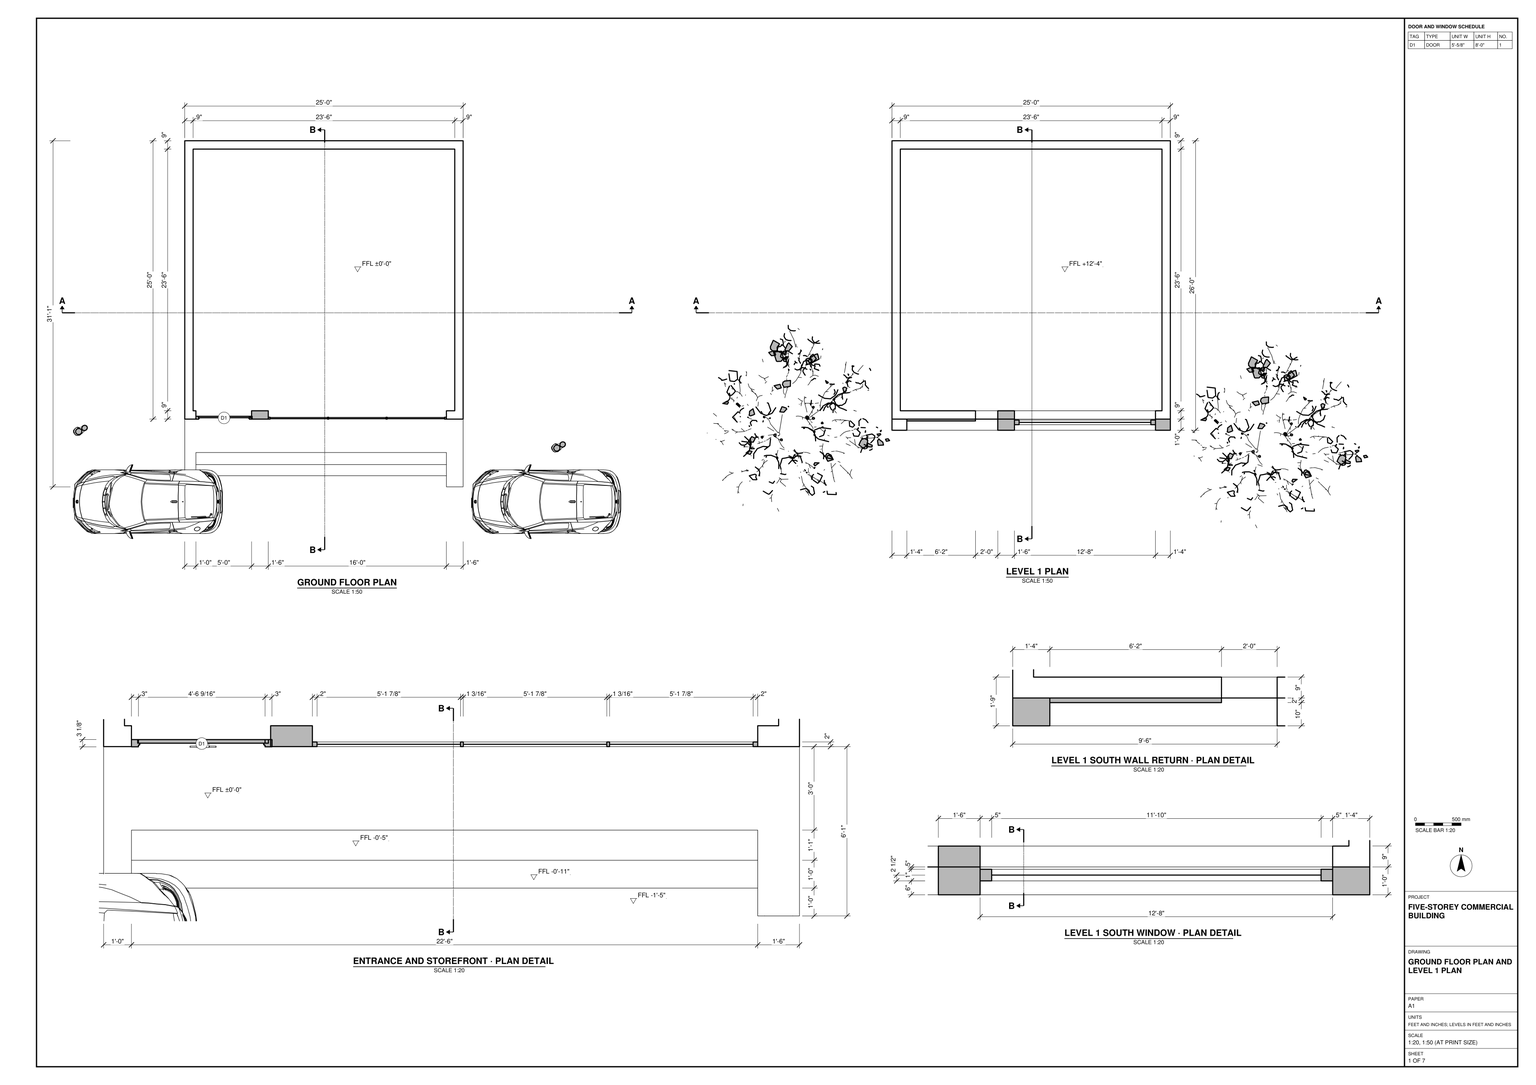
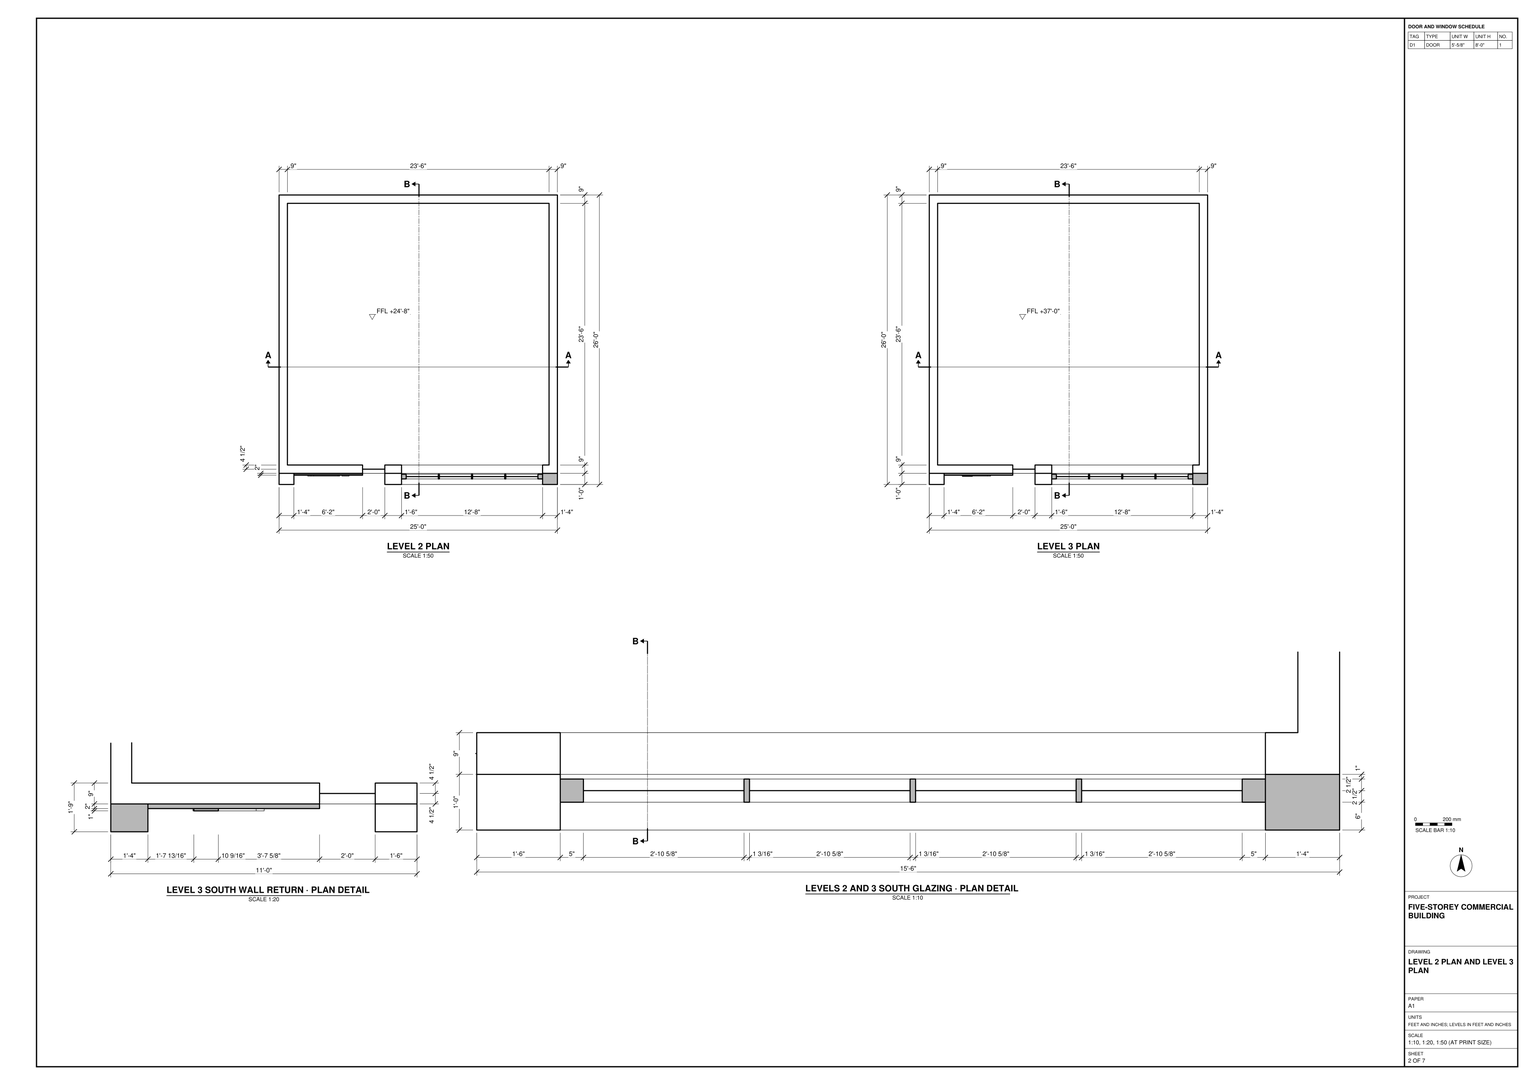
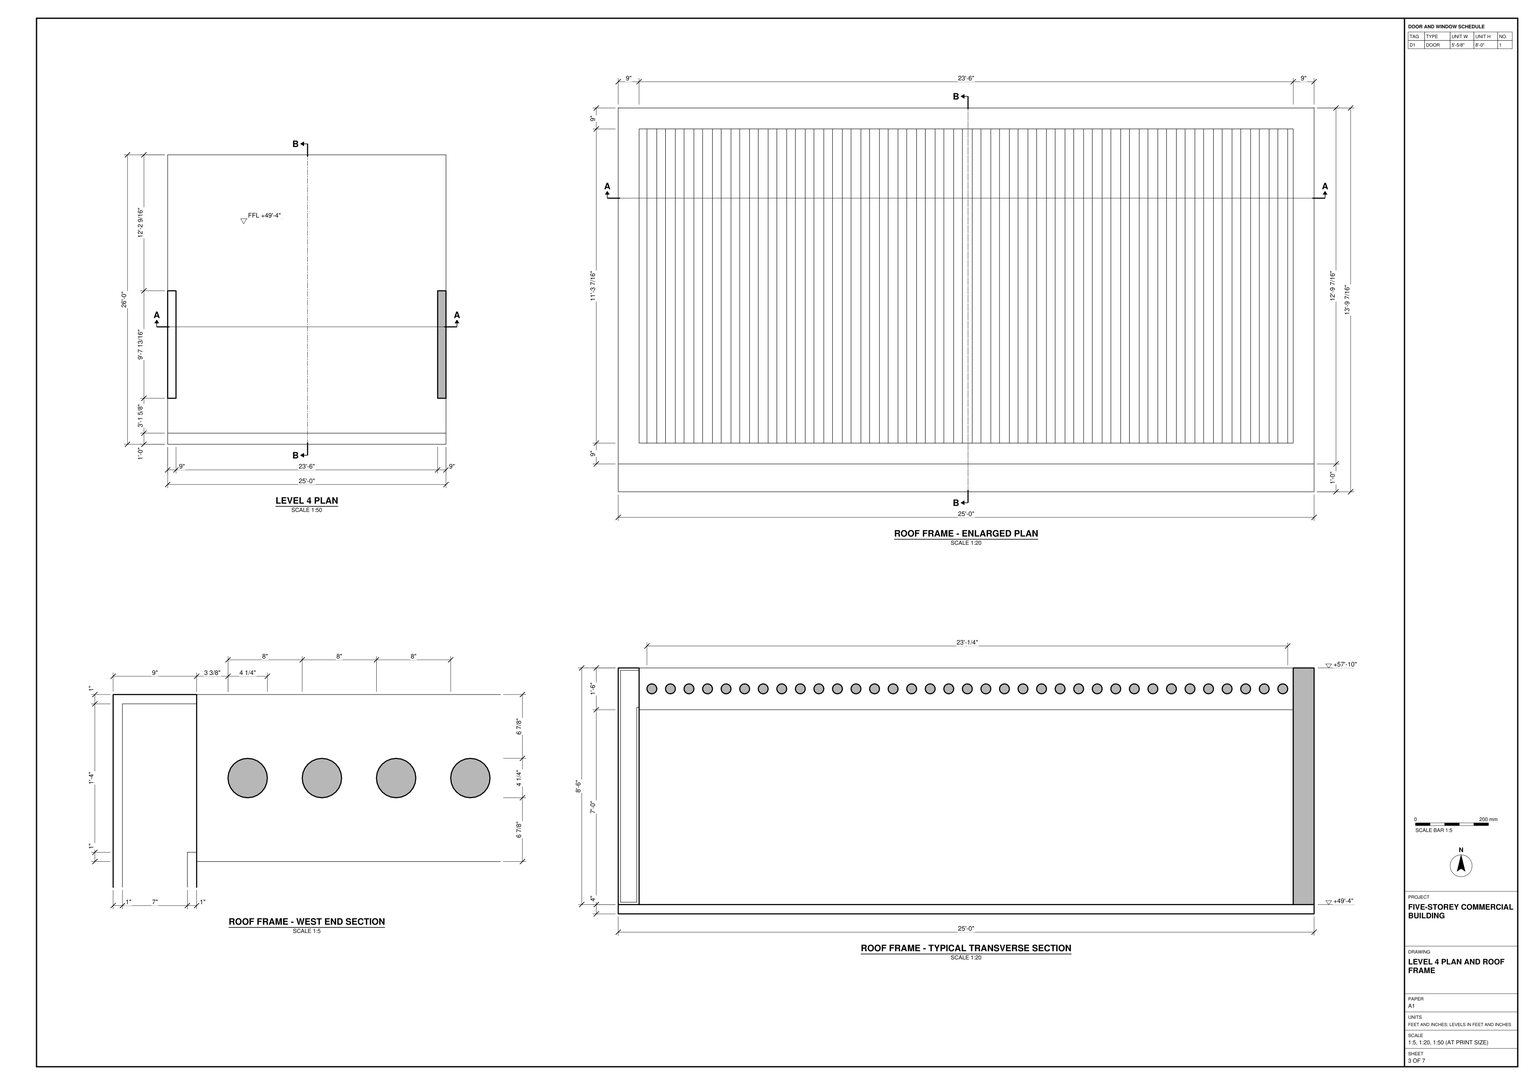
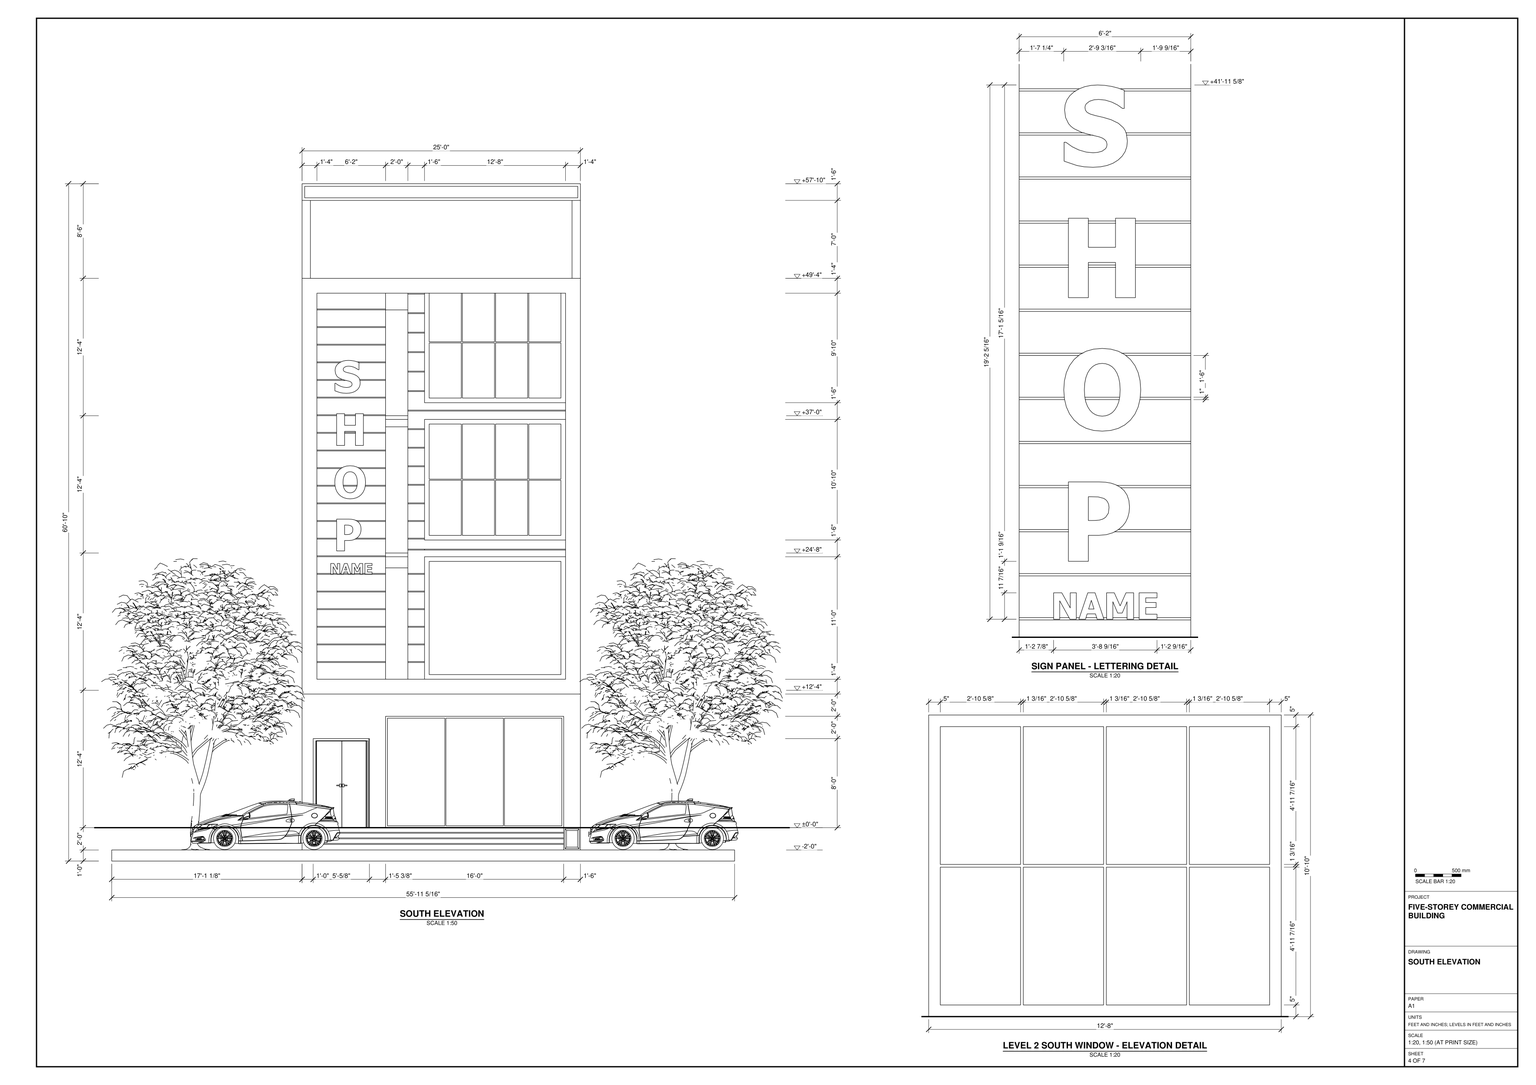
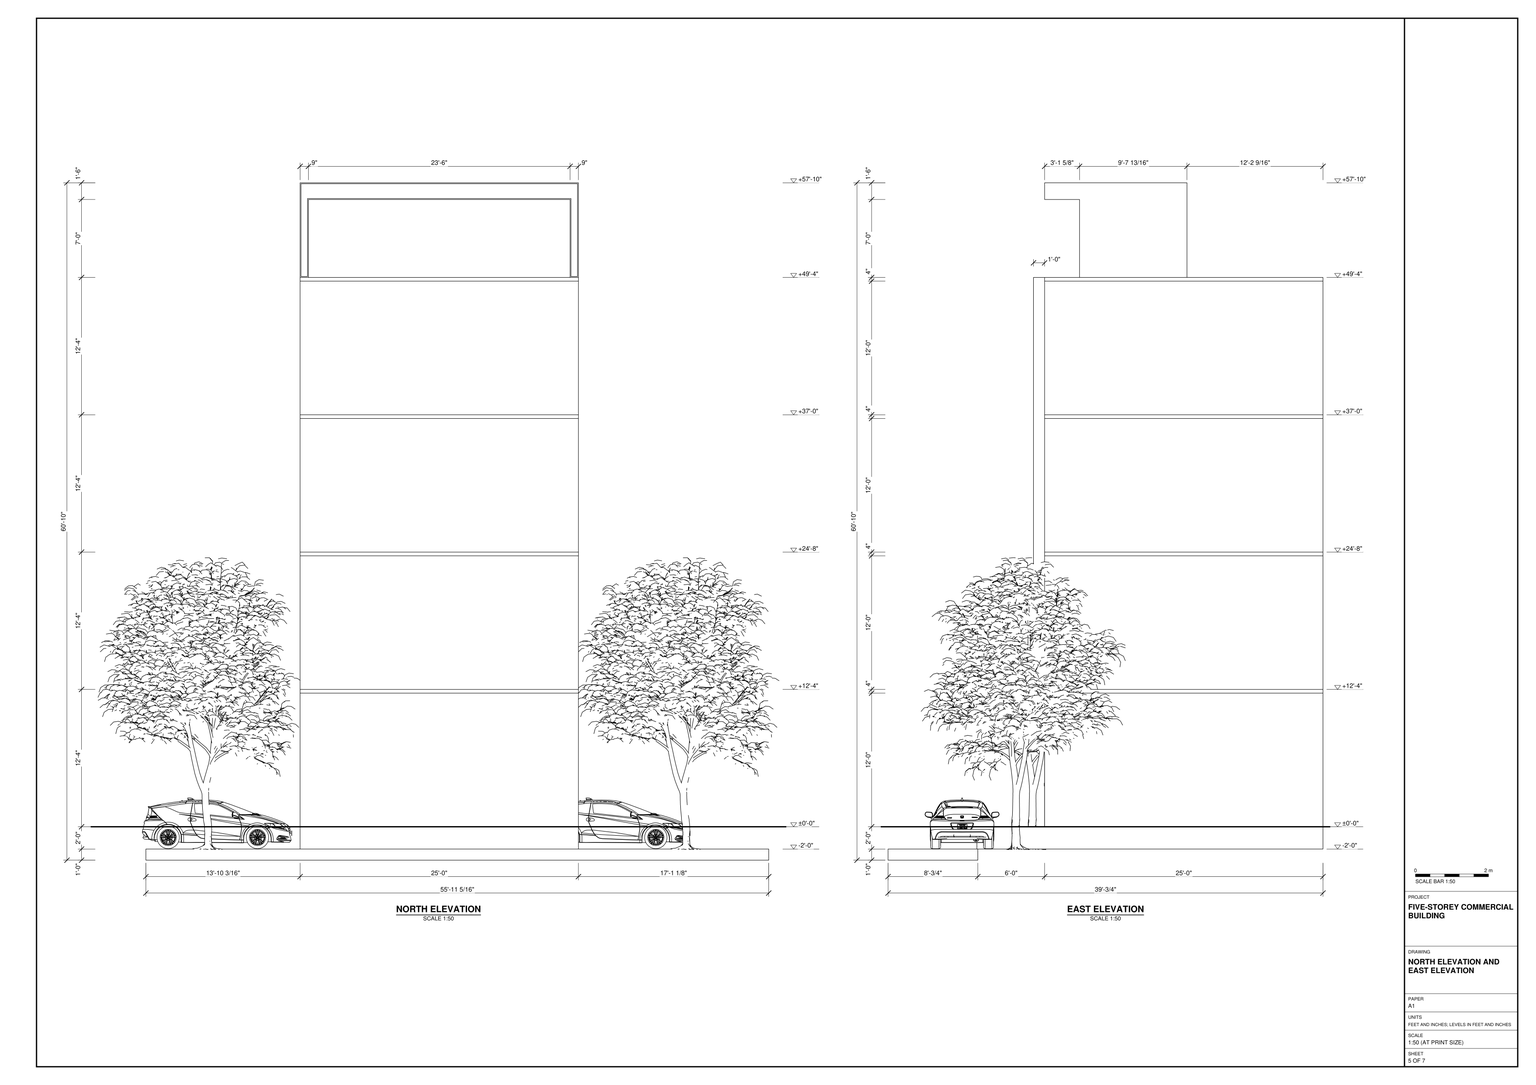
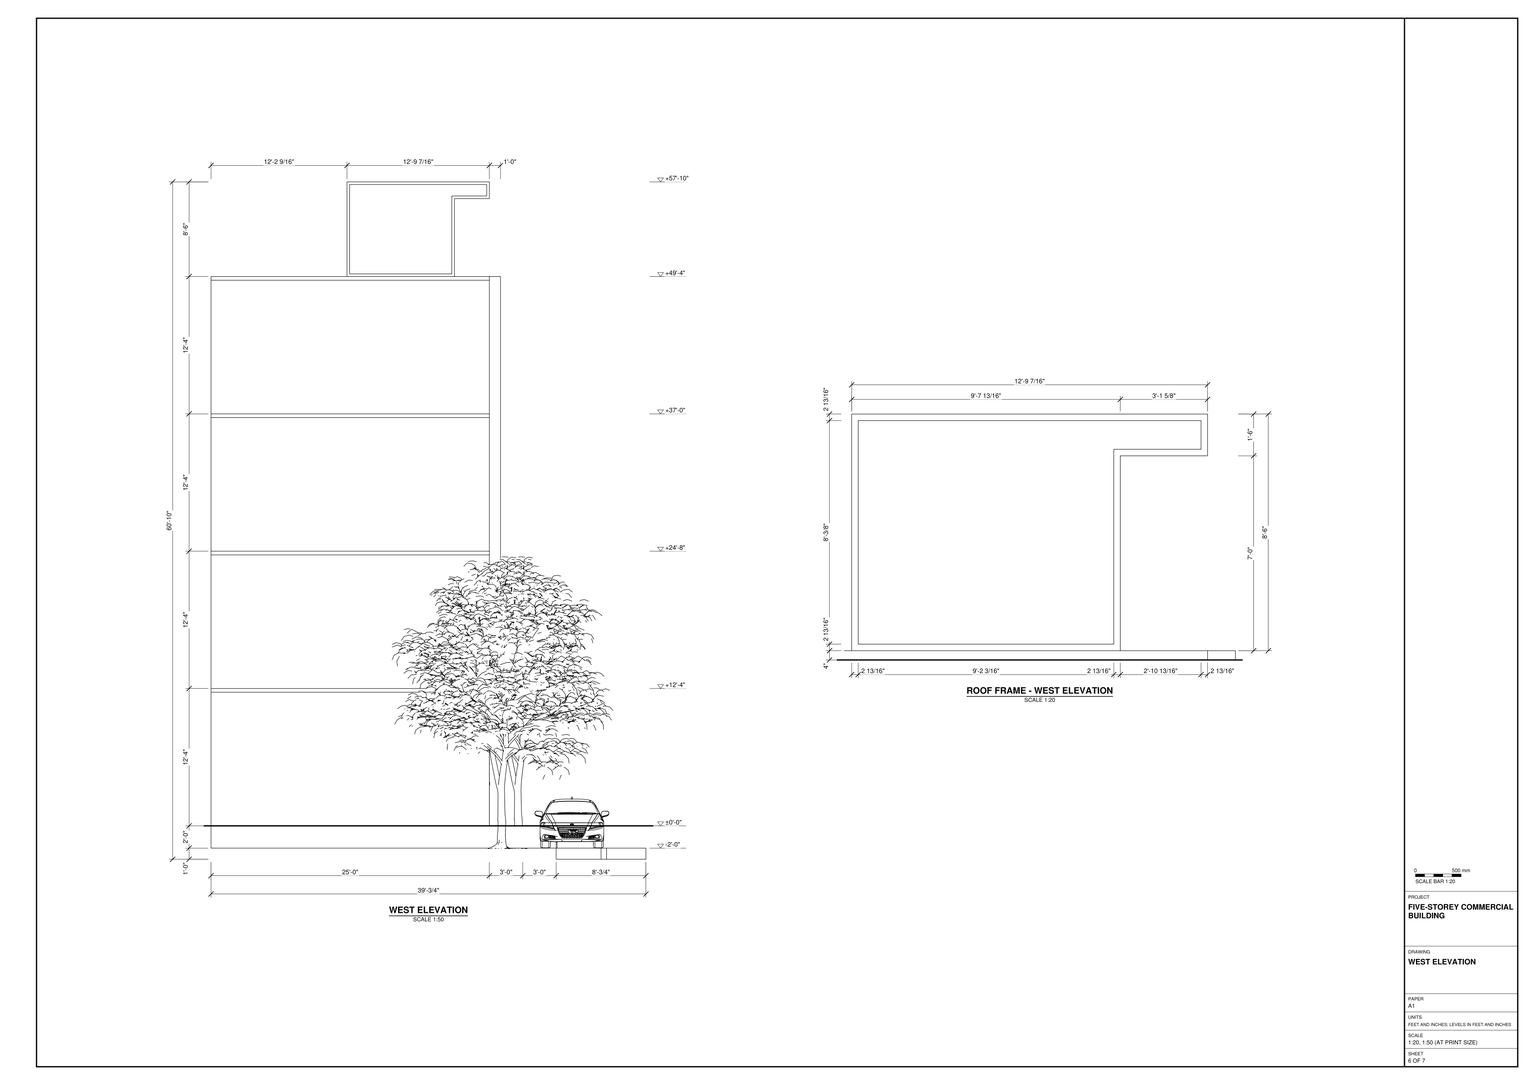
Work in feet and inches in SketchUp. Use task_files/diagram_01.pdf to model the building and its immediate surroundings. The complete model measures 61'-2" along X, 39'-3/4" along Y and 60'-10" along Z. These are the overall extents, not the dimensions of the building footprint. Set the finished floor levels at ±0'-0", +12'-4", +24'-8", +37'-0" and +49'-4".

Start with the 25'-0" square ground-floor plan. Model the floor slabs and perimeter walls with their thicknesses as drawn, keeping the floor areas open as shown. On the south side, form the wide entrance steps and landing. Place the double entrance door toward the left of the storefront and the longer run of framed glazing to its right. On the floors above, follow the plan details for the short south wall return, piers and window bays. Distinguish the long window on level 1 from the glazing divided by vertical mullions on levels 2 and 3.

Model level 4 as a deck with the raised roof frame over only part of it. Use the enlarged plan for the frame footprint and the transverse section for the side supports and regularly spaced round members. Place the parked cars near the front approach and the trees to either side as shown. Decor and loose items may be represented by any suitable library components.

Keep walls, slabs, the roof frame and each furniture or joinery piece as separate groups or components, and use components for repeated parts. Save one SketchUp model as output_files/five_storey_building_with_storefront_and_roof_frame.skp.

# SketchUp Ruby script. Lengths in inches.
U = 1.inch
M = Sketchup.active_model
def pt(a) = Geom::Point3d.new(a.map { |v| v * U })
def face(e, loops, mat)
  f = e.add_face(loops[0].map { |a| pt(a) })
  loops[1..].each { |l| e.add_face(l.map { |a| pt(a) }).erase! }
  f.material = f.back_material = mat if mat
  f
end
# faces: each face lists its corners as indices into pts; further lists are holes
def faces(e, pts, list, mat = nil) = list.each { |f| face(e, (f[0].is_a?(Array) ? f : [f]).map { |l| l.map { |i| pts[i] } }, mat) }
# xy, xz, yz: faces in a plane at the given z, y or x. An outline is a flat list of corners, or four numbers for a rectangle; further outlines are holes
def ring(l) = l.size == 4 ? [[l[0], l[1]], [l[2], l[1]], [l[2], l[3]], [l[0], l[3]]] : l.each_slice(2).to_a
def flat(e, list, mat, &to3) = list.each { |f| face(e, (f[0].is_a?(Array) ? f : [f]).map { |l| ring(l).map { |u, v| to3.(u, v) } }, mat) }
def xy(e, z, list, mat = nil) = flat(e, list, mat) { |x, y| [x, y, z] }
def xz(e, y, list, mat = nil) = flat(e, list, mat) { |x, z| [x, y, z] }
def yz(e, x, list, mat = nil) = flat(e, list, mat) { |y, z| [x, y, z] }
def lines(e, pts, list) = list.each { |a, b| e.add_line(pt(pts[a]), pt(pts[b])) }
# prism: a flat outline (further loops are holes) pulled along v
def prism(e, loops, v, mat = nil)
  f = face(e, loops, mat); d = Geom::Vector3d.new(v.map { |x| x * U })
  f.pushpull(f.normal.samedirection?(d) ? d.length : -d.length)
end
def box(e, o, s, mat = nil) = prism(e, [[o, [o[0] + s[0], o[1], o[2]], [o[0] + s[0], o[1] + s[1], o[2]], [o[0], o[1] + s[1], o[2]]]], [0, 0, s[2]], mat)
def at(x, y, z, deg = 0) = Geom::Transformation.translation(pt([x, y, z])) * Geom::Transformation.rotation(ORIGIN, Z_AXIS, deg.degrees)
def axes(o, x, y, z) = Geom::Transformation.new([*x, 0, *y, 0, *z, 0, *pt(o).to_a, 1])
def part(name) = M.definitions.add(name)
# library, detail: a bought-in or finely detailed component or shape, given as its bounding box
def library(name, o, s) = part(name).tap { |d| box(d.entities, o, s) }
def detail(e, o, s) = box(e.add_group.entities, o, s)
def put(e, d, t, mat = nil) = e.add_instance(d, t).tap { |i| i.material = mat if mat }
def group(e, t, mat = nil) = e.add_group.tap { |g| g.transformation = t; g.material = mat if mat }.entities
root = M.entities
M.materials.add("AM171_024").color = [90, 82, 72]
M.materials.add("AM171_1").color = [185, 198, 172]
M.materials.add("[Color L05]").color = [255, 0, 127]
M.materials.add("[Color M00]").color = [255, 255, 255]
M.materials.add("[Color M02]").color = [198, 198, 198]
M.materials.add("[Color M03]").color = [170, 170, 170]
M.materials.add("[Color M06]").color = [86, 86, 86]
M.materials.add("[Color M07]").color = [58, 58, 58]
M.materials.add("[Color M08]").color = [30, 30, 30]
M.materials.add("[Color M09]").color = [0, 0, 0]
M.materials.add("[Color_B21]").color = [51, 12, 0]
M.materials.add("[Color_L25]").color = [117, 101, 92]
M.materials.add("[Marble Carrara Floor Tile]").color = [204, 208, 219]
M.materials.add("[Marble Carrara Gold Floor Tile]").color = [225, 223, 217]
M.materials.add("[Translucent Glass Gray]").color = [128, 128, 128]
M.materials["[Translucent Glass Gray]"].alpha = 0.5
c1 = library("S H O P",[1.54,0,0],[33.17,205.33,1])
c2 = part("Door frame")
xy(c2.entities,0,[[0,0,0,3.9375,1.97,3.9375,1.97,1.97,2.36,1.97,2.36,1.18,2.17,1.18,2.17,0.85,1.97,0.85,1.97,0],[37.73,0,37.73,0.85,37.53,0.85,37.53,1.18,37.34,1.18,37.34,1.97,37.73,1.97,37.73,3.9375,39.7,3.9375,39.7,0]])
xy(c2.entities,82.45,[[2.36,1.18,37.34,1.97]])
xy(c2.entities,82.64,[[2.17,0.85,37.53,1.18]])
xy(c2.entities,82.84,[[1.97,0,37.73,0.85],[1.97,1.97,37.73,3.9375]])
xy(c2.entities,84.81,[[0,0,39.7,3.9375]],"[Color_B21]")
xz(c2.entities,0,[[0,0,1.97,0,1.97,82.84,37.73,82.84,37.73,0,39.7,0,39.7,84.81,0,84.81]],"[Color_L25]")
xz(c2.entities,0.85,[[1.97,0,2.17,0,2.17,82.64,37.53,82.64,37.53,0,37.73,0,37.73,82.84,1.97,82.84]],"[Color_L25]")
xz(c2.entities,1.18,[[2.17,0,2.36,0,2.36,82.45,37.34,82.45,37.34,0,37.53,0,37.53,82.64,2.17,82.64]],"[Color_B21]")
xz(c2.entities,1.97,[[1.97,0,1.97,82.84,37.73,82.84,37.73,0,37.34,0,37.34,82.45,2.36,82.45,2.36,0]])
xz(c2.entities,3.9375,[[0,0,0,84.81,39.7,84.81,39.7,0,37.73,0,37.73,82.84,1.97,82.84,1.97,0]],"[Color_B21]")
yz(c2.entities,0,[[0,0,3.9375,84.81]],"[Color_B21]")
yz(c2.entities,1.97,[[1.97,0,3.9375,82.84]])
yz(c2.entities,1.97,[[0,0,0.85,82.84]],"[Color_L25]")
yz(c2.entities,2.17,[[0.85,0,1.18,82.64]],"[Color_L25]")
yz(c2.entities,2.36,[[1.18,0,1.97,82.45]],"[Color_B21]")
yz(c2.entities,37.34,[[1.18,0,1.97,82.45]],"[Color_B21]")
yz(c2.entities,37.53,[[0.85,0,1.18,82.64]],"[Color_L25]")
yz(c2.entities,37.73,[[1.97,0,3.9375,82.84]])
yz(c2.entities,37.73,[[0,0,0.85,82.84]],"[Color_L25]")
yz(c2.entities,39.7,[[0,0,3.9375,84.81]],"[Color_B21]")
p = [[2.13,0.01,0],[2.13,0.01,82.68],[37.57,0.01,82.68],[37.57,0.01,0]]
lines(c2.entities,p,[[0,1],[1,2],[2,3]])
c3 = part("Group\#13")
xy(c3.entities,0,[[0,2.36,35.76,4.33]])
xy(c3.entities,38.8,[[1.3,0,1.36,2.36],[1.36,0,3.29,2.36]],"[Color_L25]")
xy(c3.entities,39.63,[[3.29,0.09,3.54,0.79]],"[Color_L25]")
xy(c3.entities,39.85,[[3.54,0.09,7.14,0.79]],"[Color_L25]")
xy(c3.entities,39.86,[[7.15,0.09,7.16,0.79]],"[Color_L25]")
xy(c3.entities,40.55,[[7.15,0.09,7.17,0.79]],"[Color_L25]")
xy(c3.entities,40.5625,[[3.53,0.09,7.11,0.79],[7.11,0.09,7.125,0.79]],"[Color_L25]")
xy(c3.entities,40.8125,[[3.29,0.09,3.53,0.79]],"[Color_L25]")
xy(c3.entities,41.55,[[1.35,0,1.41,2.36],[1.41,0,3.29,2.36]],"[Color_L25]")
xy(c3.entities,82.84,[[0,2.36,35.76,4.33]])
xz(c3.entities,0,[[1.3,38.8,3.29,38.8,3.29,41.55,1.35,41.55,1.28,41.54,1.23,41.52,1.17,41.49,1.07,41.41,1.03,41.37,0.99,41.31,0.97,41.26,0.95,41.2,0.93,41.08,0.93,39.17,0.95,39.11,0.96,39.0625,0.99,39.01,1.02,38.96,1.06,38.92,1.1,38.89,1.14,38.85,1.19,38.83,1.25,38.8125]],"[Color_L25]")
xz(c3.entities,0.09,[[3.29,39.63,3.54,39.63,3.54,39.85,7.14,39.85,7.15,39.86,7.16,39.86,7.18,39.87,7.1875,39.875,7.2,39.88,7.21,39.89,7.22,39.91,7.22,39.92,7.23,39.93,7.23,40.47,7.22,40.49,7.2,40.51,7.19,40.53,7.17,40.55,7.15,40.55,7.14,40.56,7.125,40.5625,3.53,40.5625,3.53,40.8125,3.29,40.8125]],"[Color_L25]")
xz(c3.entities,0.79,[[3.29,39.63,3.29,40.8125,3.53,40.8125,3.53,40.5625,7.125,40.5625,7.14,40.56,7.15,40.55,7.17,40.55,7.19,40.53,7.2,40.51,7.22,40.49,7.23,40.47,7.23,39.93,7.22,39.92,7.22,39.91,7.21,39.89,7.2,39.88,7.1875,39.875,7.18,39.87,7.16,39.86,7.15,39.86,7.14,39.85,3.54,39.85,3.54,39.63]],"[Color_L25]")
xz(c3.entities,2.36,[[[0,0,35.76,82.84],[0.93,38.8,3.29,41.55]],[0.93,38.8,1.36,38.8,1.3,38.8,1.25,38.8125,1.19,38.83,1.14,38.85,1.1,38.89,1.06,38.92,1.02,38.96,0.99,39.01,0.96,39.0625,0.95,39.11,0.93,39.17,0.93,39.22],[0.93,41.08,0.95,41.2,0.97,41.26,0.99,41.31,1.03,41.37,1.07,41.41,1.17,41.49,1.23,41.52,1.28,41.54,1.35,41.55,1.41,41.55,0.93,41.55]],"[Color_L25]")
xz(c3.entities,4.33,[[0,0,35.76,82.84]])
yz(c3.entities,0,[[2.36,0,4.33,82.84]])
yz(c3.entities,0.93,[[0,39.17,2.36,39.22],[0,39.22,2.36,41.08]],"[Color_L25]")
yz(c3.entities,3.29,[[[0,38.8,2.36,41.55],[0.09,39.63,0.79,40.8125]]],"[Color_L25]")
yz(c3.entities,3.53,[[0.09,40.5625,0.79,40.8125]],"[Color_L25]")
yz(c3.entities,3.54,[[0.09,39.63,0.79,39.85]],"[Color_L25]")
yz(c3.entities,7.22,[[0.09,39.91,0.79,39.92]],"[Color_L25]")
yz(c3.entities,7.23,[[0.09,39.93,0.79,39.94],[0.09,39.94,0.79,40.4375],[0.09,40.4375,0.79,40.46],[0.09,40.46,0.79,40.47]],"[Color_L25]")
yz(c3.entities,35.76,[[2.36,0,4.33,82.84]])
p = [[1.19,0,38.83],[1.14,0,38.85],[1.14,2.36,38.85],[1.19,2.36,38.83],[1.3,0,38.8],[1.25,0,38.8125],
  [1.25,2.36,38.8125],[1.3,2.36,38.8],[1.06,0,38.92],[1.02,0,38.96],[1.02,2.36,38.96],[1.06,2.36,38.92],
  [1.1,0,38.89],[1.1,2.36,38.89],[0.99,0,39.01],[0.99,2.36,39.01],[0.96,0,39.0625],[0.96,2.36,39.0625],
  [0.95,0,39.11],[0.95,2.36,39.11],[0.93,0,39.17],[0.93,2.36,39.17],[7.15,0.09,39.86],[7.14,0.09,39.85],
  [7.14,0.79,39.85],[7.15,0.79,39.86],[7.22,0.09,39.91],[7.21,0.09,39.89],[7.21,0.79,39.89],[7.22,0.79,39.91],
  [7.2,0.09,39.88],[7.2,0.79,39.88],[7.1875,0.09,39.875],[7.1875,0.79,39.875],[7.18,0.09,39.87],[7.18,0.79,39.87],
  [7.16,0.09,39.86],[7.16,0.79,39.86],[7.23,0.09,39.93],[7.22,0.09,39.92],[7.22,0.79,39.92],[7.23,0.79,39.93],
  [7.17,0.09,40.55],[7.18,0.09,40.54],[7.18,0.79,40.54],[7.17,0.79,40.55],[7.19,0.09,40.53],[7.19,0.79,40.53],
  [7.2,0.09,40.51],[7.2,0.79,40.51],[7.21,0.09,40.5],[7.21,0.79,40.5],[7.22,0.09,40.49],[7.22,0.79,40.49],
  [7.23,0.09,40.47],[7.23,0.79,40.47],[7.125,0.09,40.5625],[7.14,0.09,40.56],[7.14,0.79,40.56],[7.125,0.79,40.5625],
  [7.15,0.09,40.55],[7.15,0.79,40.55],[0.93,0,41.08],[0.94,0,41.14],[0.94,2.36,41.14],[0.93,2.36,41.08],
  [0.95,0,41.2],[0.95,2.36,41.2],[0.97,0,41.26],[0.97,2.36,41.26],[0.99,0,41.31],[0.99,2.36,41.31],
  [1.03,0,41.37],[1.03,2.36,41.37],[1.07,0,41.41],[1.07,2.36,41.41],[1.12,0,41.45],[1.12,2.36,41.45],
  [1.17,0,41.49],[1.17,2.36,41.49],[1.23,0,41.52],[1.23,2.36,41.52],[1.28,0,41.54],[1.28,2.36,41.54],
  [1.35,0,41.55],[1.35,2.36,41.55],[0.16,0.41,0],[0.16,0.41,82.68],[35.6,0.41,82.68],[35.6,0.41,0]]
faces(c3.entities,p,[[0,1,2,3],[4,5,6,7],[5,0,3,6],[8,9,10,11],[1,12,13,2],[12,8,11,13],[9,14,15,10],[14,16,17,15],
  [16,18,19,17],[18,20,21,19],[22,23,24,25],[26,27,28,29],[27,30,31,28],[30,32,33,31],[32,34,35,33],[34,36,37,35],
  [38,39,40,41],[42,43,44,45],[43,46,47,44],[46,48,49,47],[48,50,51,49],[50,52,53,51],[52,54,55,53],[56,57,58,59],
  [57,60,61,58],[62,63,64,65],[63,66,67,64],[66,68,69,67],[68,70,71,69],[70,72,73,71],[72,74,75,73],[74,76,77,75],
  [76,78,79,77],[78,80,81,79],[80,82,83,81],[82,84,85,83]],"[Color_L25]")
lines(c3.entities,p,[[86,87],[87,88],[88,89]])
c4 = part("Elegant+door(double)")
p = [[77.86,31.43,0],[42.82,31.43,0],[38.88,31.43,0]]
lines(c4.entities,p,[[0,1],[1,2]])
put(c4.entities,c2,axes([38.88,29.47,0],[1.93222,0,0],[0,1,0],[0,0,1]),"[Color_B21]")
put(c4.entities,c3,at(77.86,29.07,0))
put(c4.entities,c3,axes([78.05,29.07,0],[-1,0,0],[0,1,0],[0,0,1]))
c5 = part("NAME")
prism(c5.entities,[[[10.96,0,0],[8.2,0,0],[3.8,7.95,0],[3.8,0,0],[1.18,0,0],[1.18,11.41,0],[4.7,11.41,0],[8.34,4.875,0],[8.34,11.41,0],[10.96,11.41,0]]],[0,0,1])
prism(c5.entities,[[[12.05,0,0],[15.9,11.41,0],[19.03,11.41,0],[22.88,0,0],[19.93,0,0],[19.22,2.33,0],[15.63,2.33,0],[14.92,0,0]],[[18.59,4.4,0],[17.43,8.16,0],[16.26,4.4,0]]],[0,0,1])
prism(c5.entities,[[[35.67,0,0],[32.82,0,0],[32.82,7.5625,0],[30.74,2.68,0],[28.79,2.68,0],[26.71,7.5625,0],[26.71,0,0],[24.02,0,0],[24.02,11.41,0],[27.32,11.41,0],[29.85,5.78,0],[32.37,11.41,0],[35.67,11.41,0]]],[0,0,1])
prism(c5.entities,[[[38.03,0,0],[38.03,11.41,0],[45.75,11.41,0],[45.75,9.23,0],[40.88,9.23,0],[40.88,7.23,0],[45.36,7.23,0],[45.36,5.06,0],[40.88,5.06,0],[40.88,2.18,0],[45.75,2.18,0],[45.75,0,0]]],[0,0,1])
c6 = library("AM171_024_Defintion",[-287.72,-290.04,-2.17],[634.47,642.61,1000])
c7 = library("AM171_024_Defintion1",[-419.22,-426.02,309.0625],[911.71,919.28,1000])
c8 = part("SG-+Cay+Via+he (1)")
g1 = group(c8.entities,at(0,0,0))
put(g1,c6,axes([0,0,0],[0.30662,0,0],[0,0.30662,0],[0,0,0.30662]),"AM171_024")
put(g1,c7,axes([0,0,0],[0.23988,0,0],[0,0.23988,0],[0,0,0.23988]),"AM171_1")
c9 = library("Untitled (1)",[-3.82,8.01,0.375],[80.04,161.09,54.88])
c10 = part("Group6\#2")
xy(c10.entities,0,[[-94,-58,-32.125,58],[-30.9375,-58,30.9375,58],[32.125,-58,94,58]])
c11 = part("Group5\#1")
prism(c11.entities,[[[96,60,0],[96,-60,0],[-96,-60,0],[-96,60,0]],[[-32.125,-58,0],[-32.125,58,0],[-94,58,0],[-94,-58,0]],[[-30.9375,58,0],[-30.9375,-58,0],[30.9375,-58,0],[30.9375,58,0]],[[32.125,-58,0],[94,-58,0],[94,58,0],[32.125,58,0]]],[0,0,2],"[Color M08]")
put(c11.entities,c10,at(0,0,1),"[Translucent Glass Gray]")
c12 = part("Group11\#2")
xy(c12.entities,0,[[-71,-61,71,61]])
c13 = part("Group10\#1")
prism(c13.entities,[[[-76,-66,0],[-76,66,0],[76,66,0],[76,-66,0]],[[71,-61,0],[71,61,0],[-71,61,0],[-71,-61,0]]],[0,0,5],"[Color M09]")
put(c13.entities,c12,at(0,0,2.5),"[Translucent Glass Gray]")
c14 = part("Group14\#2")
xy(c14.entities,0,[[-71,-60,-36.39,-0.59],[-35.2,-60,-0.59,-0.59],[0.59,-60,35.2,-0.59],[36.39,-60,71,-0.59],[-71,0.59,-36.39,60],
  [-35.2,0.59,-0.59,60],[0.59,0.59,35.2,60],[36.39,0.59,71,60]])
c15 = part("Group13\#1")
prism(c15.entities,[[[-76,-65,0],[-76,65,0],[76,65,0],[76,-65,0]],[[35.2,60,0],[0.59,60,0],[0.59,0.59,0],[35.2,0.59,0]],[[-36.39,0.59,0],[-36.39,60,0],[-71,60,0],[-71,0.59,0]],[[-71,-0.59,0],[-71,-60,0],[-36.39,-60,0],[-36.39,-0.59,0]],[[-0.59,-60,0],[-0.59,-0.59,0],[-35.2,-0.59,0],[-35.2,-60,0]],[[71,0.59,0],[71,60,0],[36.39,60,0],[36.39,0.59,0]],[[71,-0.59,0],[36.39,-0.59,0],[36.39,-60,0],[71,-60,0]],[[0.59,-0.59,0],[0.59,-60,0],[35.2,-60,0],[35.2,-0.59,0]],[[-35.2,60,0],[-35.2,0.59,0],[-0.59,0.59,0],[-0.59,60,0]]],[0,0,5],"[Color M09]")
put(c15.entities,c14,at(0,0,2.5),"[Translucent Glass Gray]")
c16 = part("Group\#11")
prism(c16.entities,[[[1.0625,0.28,0],[0.62,0.62,0],[0.28,1.0625,0],[0.07,1.57,0],[0,2.12,0],[0.07,2.67,0],[0.28,3.18,0],[0.62,3.62,0],[1.0625,3.96,0],[1.57,4.17,0],[2.12,4.24,0],[2.67,4.17,0],[3.18,3.96,0],[3.62,3.62,0],[3.96,3.18,0],[4.17,2.67,0],[4.24,2.12,0],[4.17,1.57,0],[3.96,1.0625,0],[3.62,0.62,0],[3.18,0.28,0],[2.67,0.07,0],[2.12,0,0],[1.57,0.07,0]]],[0,0,135.4375])
c17 = part("Group\#19")
box(c17.entities,[0,0,0],[270,13,1])
prism(root,[[[487.12,132.75,-24],[487.12,132.75,-12],[487.12,120.75,-12],[487.12,120.75,-18],[487.12,108.75,-18],[487.12,108.75,-24]]],[-270,0,0])
put(root,c1,axes([238.82,166.75,298.29],[1,0,0],[0,0,1],[0,-1,0]),"[Color L05]")
put(root,c4,axes([186.41,145.39,0],[0.79,0,0],[0,0.79,0],[0,0,1.13194]))
put(root,c5,axes([234.8125,166.75,273.3],[1,0,0],[0,0,1],[0,-1,0]))
put(root,c8,at(89.49,155.63,-24))
put(root,c8,at(604.79,137.8,-24))
put(root,c9,at(76.77,115.97,-24,-90))
put(root,c9,at(506.08,115.97,-24,-90))
g2 = group(root,at(205.12,168.75,0),"[Color M03]")
xy(g2,0,[[0,0,0,300,300,300,300,0,282,0,282,9,291,9,291,291,9,291,9,9,12,9,12,0],[72,0,90,9]])
xy(g2,96,[[12,0,72,9]])
xy(g2,120,[[90,0,282,9]])
xy(g2,144,[[[0,0,300,300],[9,9,291,291]]])
xz(g2,0,[[0,0,12,0,12,96,72,96,72,0,90,0,90,120,282,120,282,0,300,0,300,144,0,144]])
xz(g2,9,[[9,0,9,144,291,144,291,0,282,0,282,120,90,120,90,0,72,0,72,96,12,96,12,0]])
xz(g2,291,[[9,0,291,144]])
xz(g2,300,[[0,0,300,144]])
yz(g2,0,[[0,0,300,144]])
yz(g2,9,[[9,0,291,144]])
yz(g2,12,[[0,0,9,96]])
yz(g2,72,[[0,0,9,96]])
yz(g2,90,[[0,0,9,120]])
yz(g2,282,[[0,0,9,120]])
yz(g2,291,[[9,0,291,144]])
yz(g2,300,[[0,0,300,144]])
p = [[282,0,0],[90,0,0]]
lines(g2,p,[[0,1]])
put(g2,c11,axes([186,2,60],[1,0,0],[0,0,1],[0,-1,0]))
g3 = group(root,at(205.12,168.75,144),"[Color M03]")
box(g3,[0,0,0],[300,300,4])
g4 = group(root,at(205.12,168.75,292),"[Color M03]")
xy(g4,0,[[0,0,300,300]])
xy(g4,4,[[0,0,300,300]])
xz(g4,0,[[0,0,90,4],[114,0,300,4]])
xz(g4,0,[[90,0,114,4]],"[Color M07]")
xz(g4,300,[[0,0,300,4]])
yz(g4,0,[[0,0,300,4]])
yz(g4,300,[[0,0,300,4]])
g5 = group(root,at(205.12,168.75,148),"[Color M03]")
xy(g5,0,[[[0,0,300,300],[9,9,291,291]]])
xy(g5,12,[[90,0,114,9],[132,0,284,9]])
xy(g5,132,[[90,0,114,9]])
xy(g5,144,[[0,0,132,0,132,9,9,9,9,291,291,291,291,9,284,9,284,0,300,0,300,300,0,300]])
xz(g5,0,[[[0,0,300,0,300,144,284,144,284,12,132,12,132,144,0,144],[90,12,114,132]]],"[Color M07]")
xz(g5,0,[[90,12,114,132]],"[Translucent Glass Gray]")
xz(g5,9,[[[9,0,9,144,132,144,132,12,284,12,284,144,291,144,291,0],[90,12,114,132]]])
xz(g5,291,[[9,0,291,144]])
xz(g5,300,[[0,0,300,144]])
yz(g5,0,[[0,0,300,144]])
yz(g5,9,[[9,0,291,144]])
yz(g5,90,[[0,12,9,132]])
yz(g5,114,[[0,12,9,132]])
yz(g5,132,[[0,12,9,144]])
yz(g5,284,[[0,12,9,144]])
yz(g5,291,[[9,0,291,144]])
yz(g5,300,[[0,0,300,144]])
put(g5,c13,axes([208,-1,78],[1,0,0],[0,0,1],[0,-1,0]))
g6 = group(root,at(205.12,168.75,440),"[Color M03]")
xy(g6,0,[[0,0,300,300]])
xy(g6,4,[[0,0,300,300]])
xz(g6,0,[[0,0,90,4],[114,0,300,4]])
xz(g6,0,[[90,0,114,4]],"[Color M07]")
xz(g6,300,[[0,0,300,4]])
yz(g6,0,[[0,0,300,4]])
yz(g6,300,[[0,0,300,4]])
g7 = group(root,at(205.12,168.75,296),"[Color M03]")
xy(g7,0,[[0,0,0,300,300,300,300,0,114,0,114,9,291,9,291,291,9,291,9,9,90,9,90,0]])
xy(g7,14,[[132,0,284,9]])
xy(g7,136,[[90,0,114,4.5],[90,4.5,114,9]])
xy(g7,144,[[0,0,132,0,132,9,9,9,9,291,291,291,291,9,284,9,284,0,300,0,300,300,0,300]])
xz(g7,0,[[0,0,90,0,90,136,114,136,114,0,300,0,300,144,284,144,284,14,132,14,132,144,0,144]],"[Color M07]")
xz(g7,4.5,[[90,0,114,136],[90,148,114,284]],"[Translucent Glass Gray]")
xz(g7,9,[[9,0,9,144,132,144,132,14,284,14,284,144,291,144,291,0,114,0,114,136,90,136,90,0]])
xz(g7,291,[[9,0,291,144]])
xz(g7,300,[[0,0,300,144]])
yz(g7,0,[[0,0,300,144]])
yz(g7,9,[[9,0,291,144]])
yz(g7,90,[[0,0,4.5,136],[4.5,0,9,136]])
yz(g7,114,[[0,0,4.5,136],[4.5,0,9,136]])
yz(g7,132,[[0,14,9,144]])
yz(g7,284,[[0,14,9,144]])
yz(g7,291,[[9,0,291,144]])
yz(g7,300,[[0,0,300,144]])
p = [[284,-6,144],[132,-6,144],[132,-6,14],[284,-6,14]]
lines(g7,p,[[0,1],[2,1],[3,2],[0,3]])
put(g7,c15,axes([208,-1,79],[1,0,0],[0,0,1],[0,-1,0]))
put(g7,c15,axes([208,-1,227],[1,0,0],[0,0,1],[0,-1,0]))
g8 = group(root,at(205.12,168.75,444),"[Color M03]")
xy(g8,0,[[0,0,0,300,300,300,300,0,114,0,114,9,291,9,291,291,9,291,9,9,90,9,90,0]])
xy(g8,14,[[132,0,284,9]])
xy(g8,114,[[90,0,114,9]])
xy(g8,132,[[132,0,284,9]])
xy(g8,144,[[[0,0,300,300],[9,9,291,291]]])
xz(g8,0,[[[0,0,90,0,90,114,114,114,114,0,300,0,300,144,0,144],[132,14,284,132]]],"[Color M07]")
xz(g8,9,[[[9,0,9,144,291,144,291,0,114,0,114,114,90,114,90,0],[132,14,284,132]]])
xz(g8,291,[[9,0,291,144]])
xz(g8,300,[[0,0,300,144]])
yz(g8,0,[[0,0,300,144]])
yz(g8,9,[[9,0,291,144]])
yz(g8,90,[[0,0,9,114]])
yz(g8,114,[[0,0,9,114]])
yz(g8,132,[[0,14,9,132]])
yz(g8,284,[[0,14,9,132]])
yz(g8,291,[[9,0,291,144]])
yz(g8,300,[[0,0,300,144]])
g9 = group(root,at(205.12,168.75,588),"[Color M03]")
box(g9,[0,0,0],[300,300,4],"[Color M03]")
g10 = group(root,at(205.12,156.75,144),"[Color M03]")
prism(g10,[[[0,12,448],[300,12,448],[300,12,0],[0,12,0]],[[284,12,432],[16,12,432],[16,12,16],[284,12,16]]],[0,-12,0])
g11 = group(root,at(221.12,166.75,160),"[Color M03]")
prism(g11,[[[0,2,416],[0,2,0],[0,0,0],[0,0,18],[0,1,18],[0,1,19],[0,0,19],[0,0,37],[0,1,37],[0,1,38],[0,0,38],[0,0,56],[0,1,56],[0,1,57],[0,0,57],[0,0,75],[0,1,75],[0,1,76],[0,0,76],[0,0,94],[0,1,94],[0,1,95],[0,0,95],[0,0,113],[0,1,113],[0,1,114],[0,0,114],[0,0,132],[0,1,132],[0,1,133],[0,0,133],[0,0,151],[0,1,151],[0,1,152],[0,0,152],[0,0,170],[0,1,170],[0,1,171],[0,0,171],[0,0,189],[0,1,189],[0,1,190],[0,0,190],[0,0,208],[0,1,208],[0,1,209],[0,0,209],[0,0,227],[0,1,227],[0,1,228],[0,0,228],[0,0,246],[0,1,246],[0,1,247],[0,0,247],[0,0,265],[0,1,265],[0,1,266],[0,0,266],[0,0,284],[0,1,284],[0,1,285],[0,0,285],[0,0,303],[0,1,303],[0,1,304],[0,0,304],[0,0,322],[0,1,322],[0,1,323],[0,0,323],[0,0,341],[0,1,341],[0,1,342],[0,0,342],[0,0,360],[0,1,360],[0,1,361],[0,0,361],[0,0,379],[0,1,379],[0,1,380],[0,0,380],[0,0,398],[0,1,398],[0,1,399],[0,0,399],[0,0,416]]],[74,0,0])
g12 = group(root,at(319.12,156.75,160),"[Color M03]")
xy(g12,0,[[0,0,18,12]])
xy(g12,132,[[18,0,170,12]])
xy(g12,150,[[18,0,170,12]])
xy(g12,280,[[18,0,170,12]])
xy(g12,298,[[18,0,170,12]])
xy(g12,416,[[0,0,18,12]])
xz(g12,0,[[0,0,18,18],[0,18,18,19],[0,19,18,37],[0,37,18,38],[0,38,18,56],
  [0,56,18,57],[0,57,18,75],[0,75,18,76],[0,76,18,94],[0,94,18,95],
  [0,95,18,113],[0,113,18,114],[0,114,18,114,18,132,170,132,170,139.1875,0,139.1875],[0,139.1875,18,140.1875],[18,139.1875,170,140.1875],
  [0,140.1875,170,140.1875,170,150,18,150,18,151,0,151],[0,151,18,152],[0,152,18,170],[0,170,18,171],[0,171,18,189],
  [0,189,18,190],[0,190,18,209],[0,209,18,210],[0,210,18,229],[0,229,18,230],
  [0,230,18,249],[0,249,18,250],[0,250,18,269],[0,269,18,270],[0,270,18,270,18,280,170,280,170,289,0,289],
  [0,289,170,290],[0,290,170,290,170,298,18,298,18,310,0,310],[0,310,18,311],[0,311,18,331],[0,331,18,332],
  [0,332,18,352],[0,352,18,353],[0,353,18,373],[0,373,18,374],[0,374,18,394],
  [0,394,18,395],[0,395,18,415],[0,415,18,416]])
xz(g12,12,[[0,0,0,416,18,416,18,298,170,298,170,280,18,280,18,150,170,150,170,132,18,132,18,0]])
yz(g12,0,[[0,0,12,416]])
yz(g12,18,[[0,0,12,132],[0,150,12,280],[0,298,12,416]])
yz(g12,170,[[0,132,12,150],[0,280,12,298]])
put(root,c16,axes([217.5,313.1875,682.88],[1,0,0],[0,0,1],[0,-1,0]),"[Color M07]")
put(root,c16,axes([225.5,313.1875,682.88],[1,0,0],[0,0,1],[0,-1,0]),"[Color M07]")
put(root,c16,axes([233.5,313.1875,682.88],[1,0,0],[0,0,1],[0,-1,0]),"[Color M07]")
put(root,c16,axes([241.5,313.1875,682.88],[1,0,0],[0,0,1],[0,-1,0]),"[Color M07]")
put(root,c16,axes([249.5,313.1875,682.88],[1,0,0],[0,0,1],[0,-1,0]),"[Color M07]")
put(root,c16,axes([257.5,313.1875,682.88],[1,0,0],[0,0,1],[0,-1,0]),"[Color M07]")
put(root,c16,axes([265.5,313.1875,682.88],[1,0,0],[0,0,1],[0,-1,0]),"[Color M07]")
put(root,c16,axes([273.5,313.1875,682.88],[1,0,0],[0,0,1],[0,-1,0]),"[Color M07]")
put(root,c16,axes([281.5,313.1875,682.88],[1,0,0],[0,0,1],[0,-1,0]),"[Color M07]")
put(root,c16,axes([289.5,313.1875,682.88],[1,0,0],[0,0,1],[0,-1,0]),"[Color M07]")
put(root,c16,axes([297.5,313.1875,682.88],[1,0,0],[0,0,1],[0,-1,0]),"[Color M07]")
put(root,c16,axes([305.5,313.1875,682.88],[1,0,0],[0,0,1],[0,-1,0]),"[Color M07]")
put(root,c16,axes([313.5,313.1875,682.88],[1,0,0],[0,0,1],[0,-1,0]),"[Color M07]")
put(root,c16,axes([321.5,313.1875,682.88],[1,0,0],[0,0,1],[0,-1,0]),"[Color M07]")
put(root,c16,axes([329.5,313.1875,682.88],[1,0,0],[0,0,1],[0,-1,0]),"[Color M07]")
put(root,c16,axes([337.5,313.1875,682.88],[1,0,0],[0,0,1],[0,-1,0]),"[Color M07]")
put(root,c16,axes([345.5,313.1875,682.88],[1,0,0],[0,0,1],[0,-1,0]),"[Color M07]")
put(root,c16,axes([353.5,313.1875,682.88],[1,0,0],[0,0,1],[0,-1,0]),"[Color M07]")
put(root,c16,axes([361.5,313.1875,682.88],[1,0,0],[0,0,1],[0,-1,0]),"[Color M07]")
put(root,c16,axes([369.5,313.1875,682.88],[1,0,0],[0,0,1],[0,-1,0]),"[Color M07]")
put(root,c16,axes([377.5,313.1875,682.88],[1,0,0],[0,0,1],[0,-1,0]),"[Color M07]")
put(root,c16,axes([385.5,313.1875,682.88],[1,0,0],[0,0,1],[0,-1,0]),"[Color M07]")
put(root,c16,axes([393.5,313.1875,682.88],[1,0,0],[0,0,1],[0,-1,0]),"[Color M07]")
put(root,c16,axes([401.5,313.1875,682.88],[1,0,0],[0,0,1],[0,-1,0]),"[Color M07]")
put(root,c16,axes([409.5,313.1875,682.88],[1,0,0],[0,0,1],[0,-1,0]),"[Color M07]")
put(root,c16,axes([417.5,313.1875,682.88],[1,0,0],[0,0,1],[0,-1,0]),"[Color M07]")
put(root,c16,axes([425.5,313.1875,682.88],[1,0,0],[0,0,1],[0,-1,0]),"[Color M07]")
put(root,c16,axes([433.5,313.1875,682.88],[1,0,0],[0,0,1],[0,-1,0]),"[Color M07]")
put(root,c16,axes([441.5,313.1875,682.88],[1,0,0],[0,0,1],[0,-1,0]),"[Color M07]")
put(root,c16,axes([449.5,313.1875,682.88],[1,0,0],[0,0,1],[0,-1,0]),"[Color M07]")
put(root,c16,axes([457.5,313.1875,682.88],[1,0,0],[0,0,1],[0,-1,0]),"[Color M07]")
put(root,c16,axes([465.5,313.1875,682.88],[1,0,0],[0,0,1],[0,-1,0]),"[Color M07]")
put(root,c16,axes([473.5,313.1875,682.88],[1,0,0],[0,0,1],[0,-1,0]),"[Color M07]")
put(root,c16,axes([481.5,313.1875,682.88],[1,0,0],[0,0,1],[0,-1,0]),"[Color M07]")
put(root,c16,axes([489.5,313.1875,682.88],[1,0,0],[0,0,1],[0,-1,0]),"[Color M07]")
g13 = group(root,at(205.12,168.75,592),"[Color M06]")
xy(g13,0,[[0,37.625,9,153.4375],[291,37.625,300,153.4375]],"[Color M07]")
xy(g13,84,[[9,0,9,9,291,9,291,37.625,300,37.625,300,0],[9,144.4375,291,153.4375]],"[Color M02]")
xy(g13,84,[[0,0,9,37.625]],"[Color M07]")
xy(g13,86.81,[[9,0,297.19,1]],"[Color M02]")
xy(g13,86.81,[[2.81,0,9,1]],"[Color M06]")
xy(g13,99.19,[[2.81,0,297.19,1]],"[Color M06]")
xy(g13,102,[[[0,0,300,153.4375],[9,9,291,144.4375]]],"[Color M02]")
xz(g13,0,[[[0,84,300,102],[2.81,86.81,297.19,99.19]]],"[Color M02]")
xz(g13,1,[[2.81,86.81,297.19,99.19]],"[Color M02]")
xz(g13,9,[[9,84,291,102]],"[Color M02]")
xz(g13,37.625,[[0,0,9,84],[291,0,300,84]],"[Color M02]")
xz(g13,144.4375,[[9,84,291,102]],"[Color M02]")
xz(g13,153.4375,[[[0,0,0,102,300,102,300,0,291,0,291,84,9,84,9,0],[1,1,8,1,8,85,292,85,292,1,299,1,299,101,1,101]],[1,1,1,101,299,101,299,1,292,1,292,85,8,85,8,1]],"[Color M02]")
yz(g13,0,[[[37.625,0,37.625,84,0,84,0,102,153.4375,102,153.4375,0],[40.44,2.81,150.62,2.81,150.62,99.19,2.81,99.19,2.81,86.81,40.44,86.81]],[40.44,2.81,40.44,86.81,2.81,86.81,2.81,99.19,150.62,99.19,150.62,2.81]],"[Color M02]")
yz(g13,2.81,[[0,86.81,1,99.19]],"[Color M06]")
yz(g13,9,[[37.625,0,153.4375,0,153.4375,84,144.4375,84,144.4375,102,9,102,9,84,37.625,84]],"[Color M02]")
yz(g13,291,[[37.625,0,37.625,84,9,84,9,102,144.4375,102,144.4375,0],[144.4375,0,153.4375,84]],"[Color M02]")
yz(g13,297.19,[[0,86.81,1,99.19]],"[Color M06]")
yz(g13,300,[[37.625,0,153.4375,0,153.4375,102,0,102,0,84,37.625,84]],"[Color M02]")
g14 = group(root,at(205.12,168.75,-24),"[Marble Carrara Gold Floor Tile]")
xy(g14,0,[[282,-73,282,-36,12,-36,12,-72,0,-72,0,300,300,300,300,-73]],"[Color M02]")
xy(g14,1.33,[[283.33,-73,298.67,-72]],"[Color M03]")
xy(g14,22.67,[[283.33,-73,298.67,-72]],"[Color M03]")
xy(g14,24,[[282,-73,300,-73,300,300,0,300,0,-72,12,-72,12,-36,282,-36]],"[Color M03]")
xz(g14,-73,[[[282,0,300,24],[283.33,1.33,298.67,22.67]],[285.03,3.03,296.97,20.97]],"[Color M03]")
xz(g14,-72,[[0,0,12,24]],"[Color M03]")
xz(g14,-36,[[12,0,282,24]])
xz(g14,300,[[0,0,300,24]],"[Color M03]")
yz(g14,0,[[-72,0,300,24]],"[Color M03]")
yz(g14,12,[[-72,0,-36,24]])
yz(g14,282,[[-73,0,-36,24]])
yz(g14,283.33,[[-73,1.33,-72,22.67]],"[Color M03]")
yz(g14,298.67,[[-73,1.33,-72,22.67]],"[Color M03]")
yz(g14,300,[[-73,0,300,24]],"[Color M03]")
p = [[296.97,-73,3.03],[285.03,-73,3.03],[283.33,-72,1.33],[298.67,-72,1.33],[283.33,-72,22.67],[285.03,-73,20.97],
  [296.97,-73,20.97],[298.67,-72,22.67]]
faces(g14,p,[[0,1,2,3],[4,2,1,5],[6,0,3,7],[7,4,5,6]],"[Color M03]")
g15 = group(root,at(217.12,120.75,-12),"[Marble Carrara Gold Floor Tile]")
box(g15,[0,0,0],[270,12,6])
g16 = group(root,at(217.12,108.75,-18),"[Marble Carrara Gold Floor Tile]")
box(g16,[0,0,0],[270,12,6])
g17 = group(root,at(217.12,96.75,-24),"[Marble Carrara Gold Floor Tile]")
box(g17,[0,0,0],[270,12,6])
put(root,c17,at(217.12,119.75,-6),"[Marble Carrara Floor Tile]")
put(root,c17,at(217.12,107.75,-12),"[Marble Carrara Floor Tile]")
put(root,c17,at(217.12,95.75,-18),"[Marble Carrara Floor Tile]")
g18 = group(root,at(0,0,-24))
xy(g18,-12,[[[0,0,0,42.375,61.95,42.375,61.95,48.375,0,48.375,0,96.75,671.31,96.75,671.31,0],[517.125,42.375,579.07,48.375],[86.1875,42.375,148.14,48.375],[172.375,42.375,234.32,48.375],[258.5625,42.375,320.51,48.375],[344.75,42.375,406.7,48.375],[430.9375,42.375,492.89,48.375],[603.3125,42.375,665.26,48.375]]],"[Color M08]")
xy(g18,0,[[0,42.375,61.95,48.375],[86.1875,42.375,148.14,48.375],[172.375,42.375,234.32,48.375],[258.5625,42.375,320.51,48.375],[344.75,42.375,406.7,48.375],
  [430.9375,42.375,492.89,48.375],[517.125,42.375,579.07,48.375],[603.3125,42.375,665.26,48.375]],"[Color M00]")
xy(g18,0,[[[0,0,0,42.375,61.95,42.375,61.95,48.375,0,48.375,0,96.75,671.31,96.75,671.31,0],[517.125,42.375,579.07,48.375],[172.375,42.375,234.32,48.375],[86.1875,42.375,148.14,48.375],[344.75,42.375,406.7,48.375],[430.9375,42.375,492.89,48.375],[258.5625,42.375,320.51,48.375],[603.3125,42.375,665.26,48.375]]],"[Color M09]")
xz(g18,0,[[0,-12,671.31,0]],"[Color M08]")
xz(g18,42.375,[[0,-12,61.95,0],[86.1875,-12,148.14,0],[172.375,-12,234.32,0],[258.5625,-12,320.51,0],[344.75,-12,406.7,0],
  [430.9375,-12,492.89,0],[517.125,-12,579.07,0],[603.3125,-12,665.26,0]],"[Color M08]")
xz(g18,48.375,[[0,-12,61.95,0],[86.1875,-12,148.14,0],[172.375,-12,234.32,0],[258.5625,-12,320.51,0],[344.75,-12,406.7,0],
  [430.9375,-12,492.89,0],[517.125,-12,579.07,0],[603.3125,-12,665.26,0]],"[Color M08]")
xz(g18,96.75,[[0,-12,671.31,0]],"[Color M08]")
yz(g18,0,[[0,-12,42.375,0],[48.375,-12,96.75,0]],"[Color M08]")
yz(g18,61.95,[[42.375,-12,48.375,0]],"[Color M08]")
yz(g18,86.1875,[[42.375,-12,48.375,0]],"[Color M08]")
yz(g18,148.14,[[42.375,-12,48.375,0]],"[Color M08]")
yz(g18,172.375,[[42.375,-12,48.375,0]],"[Color M08]")
yz(g18,234.32,[[42.375,-12,48.375,0]],"[Color M08]")
yz(g18,258.5625,[[42.375,-12,48.375,0]],"[Color M08]")
yz(g18,320.51,[[42.375,-12,48.375,0]],"[Color M08]")
yz(g18,344.75,[[42.375,-12,48.375,0]],"[Color M08]")
yz(g18,406.7,[[42.375,-12,48.375,0]],"[Color M08]")
yz(g18,430.9375,[[42.375,-12,48.375,0]],"[Color M08]")
yz(g18,492.89,[[42.375,-12,48.375,0]],"[Color M08]")
yz(g18,517.125,[[42.375,-12,48.375,0]],"[Color M08]")
yz(g18,579.07,[[42.375,-12,48.375,0]],"[Color M08]")
yz(g18,603.3125,[[42.375,-12,48.375,0]],"[Color M08]")
yz(g18,665.26,[[42.375,-12,48.375,0]],"[Color M08]")
yz(g18,671.31,[[0,-12,96.75,0]],"[Color M08]")
